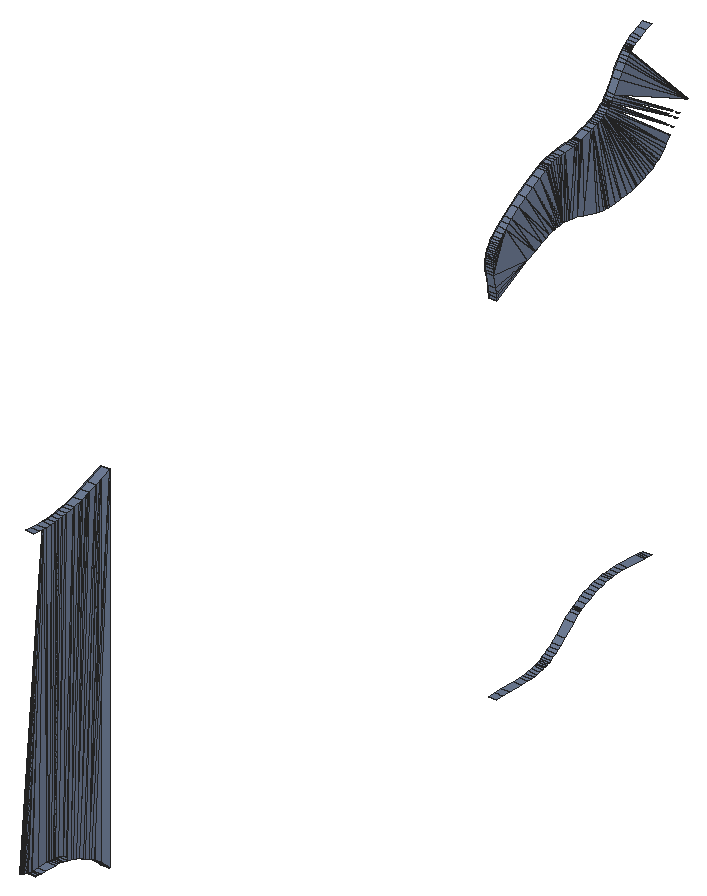
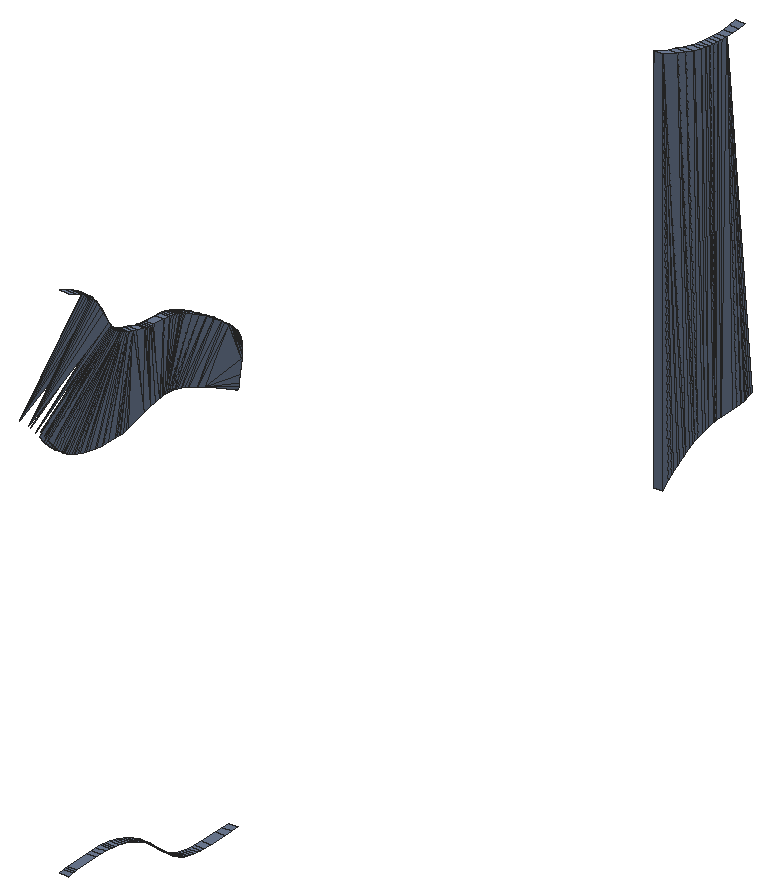
# SketchUp Ruby script. Lengths in inches.
U = 1.inch
M = Sketchup.active_model
def pt(a) = Geom::Point3d.new(a.map { |v| v * U })
def face(e, loops, mat)
  f = e.add_face(loops[0].map { |a| pt(a) })
  loops[1..].each { |l| e.add_face(l.map { |a| pt(a) }).erase! }
  f.material = f.back_material = mat if mat
  f
end
# faces: each face lists its corners as indices into pts; further lists are holes
def faces(e, pts, list, mat = nil) = list.each { |f| face(e, (f[0].is_a?(Array) ? f : [f]).map { |l| l.map { |i| pts[i] } }, mat) }
# xy, xz, yz: faces in a plane at the given z, y or x. An outline is a flat list of corners, or four numbers for a rectangle; further outlines are holes
def ring(l) = l.size == 4 ? [[l[0], l[1]], [l[2], l[1]], [l[2], l[3]], [l[0], l[3]]] : l.each_slice(2).to_a
def flat(e, list, mat, &to3) = list.each { |f| face(e, (f[0].is_a?(Array) ? f : [f]).map { |l| ring(l).map { |u, v| to3.(u, v) } }, mat) }
def xy(e, z, list, mat = nil) = flat(e, list, mat) { |x, y| [x, y, z] }
def xz(e, y, list, mat = nil) = flat(e, list, mat) { |x, z| [x, y, z] }
def yz(e, x, list, mat = nil) = flat(e, list, mat) { |y, z| [x, y, z] }
def lines(e, pts, list) = list.each { |a, b| e.add_line(pt(pts[a]), pt(pts[b])) }
# prism: a flat outline (further loops are holes) pulled along v
def prism(e, loops, v, mat = nil)
  f = face(e, loops, mat); d = Geom::Vector3d.new(v.map { |x| x * U })
  f.pushpull(f.normal.samedirection?(d) ? d.length : -d.length)
end
def box(e, o, s, mat = nil) = prism(e, [[o, [o[0] + s[0], o[1], o[2]], [o[0] + s[0], o[1] + s[1], o[2]], [o[0], o[1] + s[1], o[2]]]], [0, 0, s[2]], mat)
def at(x, y, z, deg = 0) = Geom::Transformation.translation(pt([x, y, z])) * Geom::Transformation.rotation(ORIGIN, Z_AXIS, deg.degrees)
def axes(o, x, y, z) = Geom::Transformation.new([*x, 0, *y, 0, *z, 0, *pt(o).to_a, 1])
def part(name) = M.definitions.add(name)
# library, detail: a bought-in or finely detailed component or shape, given as its bounding box
def library(name, o, s) = part(name).tap { |d| box(d.entities, o, s) }
def detail(e, o, s) = box(e.add_group.entities, o, s)
def put(e, d, t, mat = nil) = e.add_instance(d, t).tap { |i| i.material = mat if mat }
def group(e, t, mat = nil) = e.add_group.tap { |g| g.transformation = t; g.material = mat if mat }.entities
root = M.entities
M.materials.add("3D66_SU_1584934530605_002").color = [112, 126, 151]
xy(root,52,[[122.5,312.65,123.07,313.02],[122.5,313.02,123.07,313.4]],"3D66_SU_1584934530605_002")
xy(root,74.33,[[122.5,311.62,123.07,311.75],[122.5,311.75,123.07,311.88]],"3D66_SU_1584934530605_002")
xy(root,75.08,[[122.5,307.875,123.07,308.02]],"3D66_SU_1584934530605_002")
xz(root,269.95,[[122.5,53.02,123.07,77.01]],"3D66_SU_1584934530605_002")
xz(root,302.18,[[122.5,74.85,123.07,75.04],[122.5,75.04,123.07,75.14]],"3D66_SU_1584934530605_002")
yz(root,122.5,[[269.95,53.02,269.54,53.4,269.95,77.01],[269.54,53.4,269.33,53.58,269.95,77.01],[269.33,53.58,269.11,53.75,269.95,77.01],[269.11,53.75,268.89,53.9,269.95,77.01],[268.89,53.9,268.66,54.05,269.95,77.01],
  [268.66,54.05,268.43,54.2,269.95,77.01],[268.43,54.2,268.19,54.33,269.95,77.01],[268.19,54.33,267.95,54.45,268.79,76.57],[268.19,54.33,268.79,76.57,269.95,77.01],[267.95,54.45,267.72,54.5625,268.79,76.57],
  [267.72,54.5625,267.48,54.67,268.79,76.57],[267.48,54.67,267.23,54.76,268.2,76.37],[267.48,54.67,268.2,76.37,268.79,76.57],[267.23,54.76,266.98,54.85,267.6,76.18],[267.23,54.76,267.6,76.18,268.2,76.37],
  [266.98,54.85,266.71,54.93,267.6,76.18],[266.71,54.93,266.43,55,266.99,76.03],[266.71,54.93,266.99,76.03,267.6,76.18],[266.43,55,266.13,55.07,266.68,75.97],[266.43,55,266.68,75.97,266.99,76.03],
  [266.13,55.07,266.05,55.09,266.37,75.91],[266.13,55.07,266.37,75.91,266.68,75.97],[266.05,55.09,265.97,55.1,266.37,75.91],[265.97,55.1,265.79,55.12,266.05,75.87],[265.97,55.1,266.05,75.87,266.37,75.91],
  [265.79,55.12,265.61,55.13,265.72,75.84],[265.79,55.12,265.72,75.84,266.05,75.87],[265.61,55.13,265.4,75.82,265.72,75.84],[265.61,55.13,265.43,55.14,265.4,75.82],[265.43,55.14,264.64,55.15,265.06,75.81],
  [265.43,55.14,265.06,75.81,265.4,75.82],[264.64,55.15,264.24,55.16,265.06,75.81],[264.24,55.16,264.05,55.18,265.06,75.81],[264.05,55.18,263.86,55.2,265.06,75.81],[263.86,55.2,263.76,55.22,265.06,75.81],
  [263.76,55.22,263.67,55.24,265.06,75.81],[263.67,55.24,263.58,55.26,265.06,75.81],[263.58,55.26,263.49,55.28,265.06,75.81],[263.49,55.28,263.41,55.31,265.06,75.81],[263.41,55.31,263.32,55.34,265.06,75.81],
  [263.32,55.34,263.24,55.37,265.06,75.81],[263.24,55.37,263.16,55.41,265.06,75.81],[302.48,72.84,302.47,73.04,304.99,74.12],[302.47,73.04,302.45,73.24,304.99,74.12],[302.45,73.24,302.38,73.64,304.99,74.12],
  [302.38,73.64,302.22,74.45,304.99,74.12],[304.99,74.12,302.22,74.45,303.24,76.8],[304.99,74.12,303.24,76.8,305.61,74.43],[311.62,74.33,310.54,79.64,311.75,74.33],[311.62,74.33,311.49,74.35,310.54,79.64],
  [311.75,74.33,310.54,79.64,311.88,74.33],[311.88,74.33,310.54,79.64,310.83,79.73],[311.88,74.33,310.83,79.73,312.39,74.34],[312.39,74.34,310.83,79.73,310.97,79.78],[312.39,74.34,310.97,79.78,312.89,74.375],
  [311.49,74.35,311.36,74.36,310.54,79.64],[311.36,74.36,311.09,74.41,310.54,79.64],[312.89,74.375,310.97,79.78,311.11,79.84],[312.89,74.375,311.11,79.84,313.38,74.43],[311.09,74.41,310.83,74.47,310.54,79.64],
  [305.61,74.43,303.24,76.8,303.49,77],[305.61,74.43,303.49,77,303.75,77.21],[305.61,74.43,303.75,77.21,306.23,74.69],[313.38,74.43,311.11,79.84,311.24,79.9],[313.38,74.43,311.24,79.9,313.86,74.51],
  [302.22,74.45,302.2,74.65,303.01,76.6],[302.22,74.45,303.01,76.6,303.24,76.8],[310.83,74.47,309.73,74.77,310.54,79.64],[313.86,74.51,311.24,79.9,314.1,74.57],[314.1,74.57,311.24,79.9,311.375,79.97],
  [314.1,74.57,311.375,79.97,314.33,74.625],[314.33,74.625,311.375,79.97,314.56,74.6875],[302.2,74.65,302.18,74.85,302.8,76.4],[302.2,74.65,302.8,76.4,303.01,76.6],[314.56,74.6875,311.375,79.97,314.78,74.76],
  [306.23,74.69,303.75,77.21,304.33,77.6],[306.23,74.69,304.33,77.6,306.54,74.81],[314.78,74.76,311.375,79.97,315,74.84],[309.73,74.77,309.17,74.92,309.61,79.39],[309.73,74.77,309.61,79.39,310.25,79.5625],
  [309.73,74.77,310.25,79.5625,310.54,79.64],[306.54,74.81,304.33,77.6,306.84,74.9],[315,74.84,311.375,79.97,311.51,80.05],[315,74.84,311.51,80.05,315.22,74.94],[302.18,74.85,302.18,75.04,302.8,76.4],
  [306.84,74.9,304.33,77.6,304.92,77.98],[306.84,74.9,304.92,77.98,307.14,74.98],[309.17,74.92,308.88,74.98,309.27,79.32],[309.17,74.92,309.27,79.32,309.44,79.35],[309.17,74.92,309.44,79.35,309.53,79.37],
  [309.17,74.92,309.53,79.37,309.61,79.39],[315.22,74.94,311.51,80.05,315.43,75.03],[307.14,74.98,304.92,77.98,307.29,75.01],[308.88,74.98,308.6,75.03,309.1,79.3],[308.88,74.98,309.1,79.3,309.27,79.32],
  [307.29,75.01,304.92,77.98,305.51,78.32],[307.29,75.01,305.51,78.32,307.44,75.04],[308.6,75.03,308.19,79.25,308.92,79.29],[308.6,75.03,308.45,75.05,308.19,79.25],[308.6,75.03,308.92,79.29,309.1,79.3],
  [315.43,75.03,311.51,80.05,315.64,75.14],[302.18,75.04,302.18,75.14,302.625,76.2],[302.18,75.04,302.625,76.2,302.71,76.3],[302.18,75.04,302.71,76.3,302.8,76.4],[307.44,75.04,305.51,78.32,307.58,75.06],
  [308.45,75.05,308.31,75.0625,308.19,79.25],[307.58,75.06,305.51,78.32,306.07,78.62],[307.58,75.06,306.07,78.62,307.73,75.07],[308.31,75.0625,308.16,75.07,308.19,79.25],[307.73,75.07,306.07,78.62,307.875,75.08],
  [308.16,75.07,307.81,79.21,308.19,79.25],[308.16,75.07,308.02,75.08,307.81,79.21],[307.875,75.08,306.07,78.62,306.56,78.86],[307.875,75.08,306.56,78.86,306.67,78.91],[307.875,75.08,306.67,78.91,306.78,78.96],
  [307.875,75.08,306.78,78.96,306.88,79],[307.875,75.08,306.88,79,306.99,79.04],[307.875,75.08,306.99,79.04,308.02,75.08],[308.02,75.08,306.99,79.04,307.2,79.1],[308.02,75.08,307.2,79.1,307.41,79.15],
  [308.02,75.08,307.41,79.15,307.61,79.1875],[308.02,75.08,307.61,79.1875,307.81,79.21],[302.18,75.14,302.19,75.24,302.55,76.11],[302.18,75.14,302.55,76.11,302.625,76.2],[315.64,75.14,311.51,80.05,315.74,75.2],
  [315.74,75.2,311.51,80.05,315.84,75.26],[302.19,75.24,302.21,75.34,302.55,76.11],[315.84,75.26,311.51,80.05,315.93,75.33],[315.93,75.33,311.51,80.05,316.02,75.4],[302.21,75.34,302.23,75.4375,302.48,76.01],
  [302.21,75.34,302.48,76.01,302.55,76.11],[316.02,75.4,311.51,80.05,316.2,75.55],[302.23,75.4375,302.25,75.53,302.48,76.01],[302.25,75.53,302.28,75.63,302.32,75.73],[302.25,75.53,302.32,75.73,302.37,75.82],
  [302.25,75.53,302.37,75.82,302.42,75.92],[302.25,75.53,302.42,75.92,302.48,76.01],[316.2,75.55,311.51,80.05,316.36,75.71],[316.36,75.71,311.51,80.05,316.52,75.88],[316.52,75.88,311.51,80.05,316.68,76.06],
  [316.68,76.06,311.51,80.05,311.64,80.13],[316.68,76.06,311.64,80.13,311.77,80.23],[316.68,76.06,311.77,80.23,316.98,76.43],[316.98,76.43,311.77,80.23,311.9,80.33],[317.3,76.82,311.9,80.33,311.97,80.39],
  [317.3,76.82,311.97,80.39,312.03,80.45],[317.3,76.82,312.03,80.45,312.09,80.52],[317.64,77.21,312.09,80.52,312.15,80.59],[317.64,77.21,312.15,80.59,312.27,80.74],[317.82,77.41,312.27,80.74,312.38,80.9],
  [318.47,77.96,312.38,80.9,312.8,81.6],[318.47,77.96,312.8,81.6,313.02,81.97],[318.47,77.96,313.02,81.97,313.25,82.34],[318.47,77.96,313.25,82.34,313.38,82.51],[318.47,77.96,313.38,82.51,313.51,82.67],
  [318.47,77.96,313.51,82.67,313.66,82.83],[318.47,77.96,313.66,82.83,313.73,82.9]],"3D66_SU_1584934530605_002")
yz(root,123.07,[[268.66,54.05,269.95,77.01,268.43,54.2],[268.43,54.2,269.95,77.01,268.19,54.33],[268.19,54.33,268.79,76.57,267.95,54.45],[267.95,54.45,268.79,76.57,267.72,54.5625],[267.72,54.5625,268.79,76.57,267.48,54.67],
  [267.48,54.67,268.2,76.37,267.23,54.76],[267.23,54.76,267.6,76.18,266.98,54.85],[266.98,54.85,267.6,76.18,266.71,54.93],[266.71,54.93,266.99,76.03,266.43,55],[302.48,72.84,304.99,74.12,302.47,73.04],
  [302.47,73.04,304.99,74.12,302.45,73.24],[302.45,73.24,304.99,74.12,302.38,73.64],[302.38,73.64,304.99,74.12,302.22,74.45],[304.99,74.12,303.24,76.8,302.22,74.45],[304.99,74.12,305.61,74.43,303.24,76.8],
  [311.62,74.33,310.54,79.64,311.49,74.35],[311.62,74.33,311.75,74.33,310.54,79.64],[311.75,74.33,311.88,74.33,310.54,79.64],[311.88,74.33,310.83,79.73,310.54,79.64],[311.88,74.33,312.39,74.34,310.83,79.73],
  [312.39,74.34,310.97,79.78,310.83,79.73],[312.39,74.34,312.89,74.375,310.97,79.78],[311.49,74.35,310.54,79.64,311.36,74.36],[311.36,74.36,310.54,79.64,311.09,74.41],[312.89,74.375,311.11,79.84,310.97,79.78],
  [312.89,74.375,313.38,74.43,311.11,79.84],[311.09,74.41,310.54,79.64,310.83,74.47],[305.61,74.43,303.49,77,303.24,76.8],[305.61,74.43,303.75,77.21,303.49,77],[305.61,74.43,306.23,74.69,303.75,77.21],
  [313.38,74.43,311.24,79.9,311.11,79.84],[313.38,74.43,313.86,74.51,311.24,79.9],[302.22,74.45,303.01,76.6,302.2,74.65],[302.22,74.45,303.24,76.8,303.01,76.6],[310.83,74.47,310.54,79.64,309.73,74.77],
  [313.86,74.51,314.1,74.57,311.24,79.9],[314.1,74.57,311.375,79.97,311.24,79.9],[314.1,74.57,314.33,74.625,311.375,79.97],[314.33,74.625,314.56,74.6875,311.375,79.97],[302.2,74.65,302.8,76.4,302.18,74.85],
  [302.2,74.65,303.01,76.6,302.8,76.4],[314.56,74.6875,314.78,74.76,311.375,79.97],[306.23,74.69,304.33,77.6,303.75,77.21],[306.23,74.69,306.54,74.81,304.33,77.6],[314.78,74.76,315,74.84,311.375,79.97],
  [309.73,74.77,309.61,79.39,309.17,74.92],[309.73,74.77,310.25,79.5625,309.61,79.39],[309.73,74.77,310.54,79.64,310.25,79.5625],[306.54,74.81,306.84,74.9,304.33,77.6],[315,74.84,311.51,80.05,311.375,79.97],
  [315,74.84,315.22,74.94,311.51,80.05],[302.18,74.85,302.8,76.4,302.18,75.04],[306.84,74.9,304.92,77.98,304.33,77.6],[306.84,74.9,307.14,74.98,304.92,77.98],[309.17,74.92,309.27,79.32,308.88,74.98],
  [309.17,74.92,309.44,79.35,309.27,79.32],[309.17,74.92,309.53,79.37,309.44,79.35],[309.17,74.92,309.61,79.39,309.53,79.37],[315.22,74.94,315.43,75.03,311.51,80.05],[307.14,74.98,307.29,75.01,304.92,77.98],
  [308.88,74.98,309.1,79.3,308.6,75.03],[308.88,74.98,309.27,79.32,309.1,79.3],[307.29,75.01,305.51,78.32,304.92,77.98],[307.29,75.01,307.44,75.04,305.51,78.32],[308.6,75.03,308.19,79.25,308.45,75.05],
  [308.6,75.03,308.92,79.29,308.19,79.25],[308.6,75.03,309.1,79.3,308.92,79.29],[315.43,75.03,315.64,75.14,311.51,80.05],[302.18,75.04,302.625,76.2,302.18,75.14],[302.18,75.04,302.71,76.3,302.625,76.2],
  [302.18,75.04,302.8,76.4,302.71,76.3],[307.44,75.04,307.58,75.06,305.51,78.32],[308.45,75.05,308.19,79.25,308.31,75.0625],[307.58,75.06,306.07,78.62,305.51,78.32],[307.58,75.06,307.73,75.07,306.07,78.62],
  [308.31,75.0625,308.19,79.25,308.16,75.07],[307.73,75.07,307.875,75.08,306.07,78.62],[308.16,75.07,307.81,79.21,308.02,75.08],[308.16,75.07,308.19,79.25,307.81,79.21],[307.875,75.08,306.56,78.86,306.07,78.62],
  [307.875,75.08,306.67,78.91,306.56,78.86],[307.875,75.08,306.78,78.96,306.67,78.91],[307.875,75.08,306.88,79,306.78,78.96],[307.875,75.08,306.99,79.04,306.88,79],[307.875,75.08,308.02,75.08,306.99,79.04],
  [308.02,75.08,307.2,79.1,306.99,79.04],[308.02,75.08,307.41,79.15,307.2,79.1],[308.02,75.08,307.61,79.1875,307.41,79.15],[308.02,75.08,307.81,79.21,307.61,79.1875],[302.18,75.14,302.55,76.11,302.19,75.24],
  [302.18,75.14,302.625,76.2,302.55,76.11],[315.64,75.14,315.74,75.2,311.51,80.05],[315.74,75.2,315.84,75.26,311.51,80.05],[302.19,75.24,302.55,76.11,302.21,75.34],[315.84,75.26,315.93,75.33,311.51,80.05],
  [315.93,75.33,316.02,75.4,311.51,80.05],[302.21,75.34,302.48,76.01,302.23,75.4375],[302.21,75.34,302.55,76.11,302.48,76.01],[316.02,75.4,316.2,75.55,311.51,80.05],[302.23,75.4375,302.48,76.01,302.25,75.53],
  [302.25,75.53,302.32,75.73,302.28,75.63],[302.25,75.53,302.37,75.82,302.32,75.73],[302.25,75.53,302.42,75.92,302.37,75.82],[302.25,75.53,302.48,76.01,302.42,75.92],[316.2,75.55,316.36,75.71,311.51,80.05],
  [316.36,75.71,316.52,75.88,311.51,80.05],[316.52,75.88,316.68,76.06,311.51,80.05],[316.68,76.06,311.64,80.13,311.51,80.05],[316.68,76.06,311.77,80.23,311.64,80.13],[316.68,76.06,316.98,76.43,311.77,80.23],
  [316.98,76.43,311.9,80.33,311.77,80.23],[317.3,76.82,311.97,80.39,311.9,80.33],[317.3,76.82,312.03,80.45,311.97,80.39],[317.3,76.82,312.09,80.52,312.03,80.45],[317.64,77.21,312.15,80.59,312.09,80.52],
  [317.64,77.21,312.27,80.74,312.15,80.59],[317.82,77.41,312.38,80.9,312.27,80.74],[318.47,77.96,312.8,81.6,312.38,80.9],[318.47,77.96,313.02,81.97,312.8,81.6],[318.47,77.96,313.25,82.34,313.02,81.97],
  [318.47,77.96,313.38,82.51,313.25,82.34],[318.47,77.96,313.51,82.67,313.38,82.51],[318.47,77.96,313.66,82.83,313.51,82.67],[318.47,77.96,313.73,82.9,313.66,82.83]],"3D66_SU_1584934530605_002")
p = [[123.07,303,48.85],[122.5,303,48.85],[122.5,302.48,48.84],[123.07,302.48,48.84],[123.07,303.52,48.84],[122.5,303.52,48.84],
  [123.07,304.58,48.81],[122.5,304.58,48.81],[123.07,305.1,48.82],[122.5,305.1,48.82],[123.07,305.36,48.83],[122.5,305.36,48.83],
  [123.07,305.61,48.85],[122.5,305.61,48.85],[123.07,305.85,48.88],[122.5,305.85,48.88],[123.07,306.09,48.92],[122.5,306.09,48.92],
  [123.07,306.33,48.97],[122.5,306.33,48.97],[123.07,306.44,49],[122.5,306.44,49],[123.07,306.56,49.03],[122.5,306.56,49.03],
  [123.07,306.67,49.07],[122.5,306.67,49.07],[123.07,306.78,49.12],[122.5,306.78,49.12],[123.07,306.88,49.16],[122.5,306.88,49.16],
  [123.07,306.99,49.22],[122.5,306.99,49.22],[123.07,307.2,49.33],[122.5,307.2,49.33],[123.07,307.41,49.46],[122.5,307.41,49.46],
  [123.07,307.61,49.6],[122.5,307.61,49.6],[123.07,307.81,49.75],[122.5,307.81,49.75],[123.07,308.19,50.06],[122.5,308.19,50.06],
  [123.07,308.92,50.67],[122.5,308.92,50.67],[123.07,309.27,50.94],[122.5,309.27,50.94],[123.07,309.44,51.06],[122.5,309.44,51.06],
  [122.5,309.53,51.11],[123.07,309.53,51.11],[122.5,309.61,51.16],[123.07,309.61,51.16],[123.07,309.93,51.32],[122.5,309.93,51.32],
  [123.07,310.23,51.46],[122.5,310.23,51.46],[123.07,310.51,51.58],[122.5,310.51,51.58],[123.07,310.79,51.68],[122.5,310.79,51.68],
  [123.07,311.06,51.76],[122.5,311.06,51.76],[123.07,311.34,51.83],[122.5,311.34,51.83],[123.07,311.63,51.89],[122.5,311.63,51.89],
  [123.07,315.45,51.84],[122.5,315.45,51.84],[122.5,315.15,51.89],[123.07,315.15,51.89],[123.07,311.94,51.9375],[122.5,311.94,51.9375],
  [123.07,312.11,51.96],[122.5,312.11,51.96],[123.07,314.84,51.92],[122.5,314.84,51.92],[122.5,313.4,52],[123.07,313.4,52],
  [123.07,315,51.91],[122.5,315,51.91],[123.07,312.29,51.98],[122.5,312.29,51.98],[123.07,312.65,52],[122.5,312.65,52],
  [123.07,269.54,53.4],[122.5,269.54,53.4],[122.5,269.95,53.02],[123.07,269.95,53.02],[123.07,269.33,53.58],[122.5,269.33,53.58],
  [123.07,269.11,53.75],[122.5,269.11,53.75],[123.07,268.89,53.9],[122.5,268.89,53.9],[123.07,268.66,54.05],[122.5,268.66,54.05],
  [123.07,268.43,54.2],[122.5,268.43,54.2],[123.07,268.19,54.33],[122.5,268.19,54.33],[123.07,267.95,54.45],[122.5,267.95,54.45],
  [123.07,267.72,54.5625],[122.5,267.72,54.5625],[123.07,267.48,54.67],[122.5,267.48,54.67],[123.07,267.23,54.76],[122.5,267.23,54.76],
  [123.07,266.71,54.93],[122.5,266.71,54.93],[122.5,266.98,54.85],[123.07,266.98,54.85],[123.07,266.43,55],[122.5,266.43,55],
  [123.07,266.13,55.07],[122.5,266.13,55.07],[123.07,264.24,55.16],[122.5,264.24,55.16],[122.5,264.64,55.15],[123.07,264.64,55.15],
  [122.5,265.43,55.14],[123.07,265.43,55.14],[122.5,265.61,55.13],[123.07,265.61,55.13],[122.5,265.79,55.12],[123.07,265.79,55.12],
  [122.5,265.97,55.1],[123.07,265.97,55.1],[122.5,266.05,55.09],[123.07,266.05,55.09],[123.07,263.76,55.22],[122.5,263.76,55.22],
  [122.5,263.86,55.2],[123.07,263.86,55.2],[122.5,264.05,55.18],[123.07,264.05,55.18],[123.07,302.47,73.04],[122.5,302.47,73.04],
  [122.5,302.48,72.84],[123.07,302.48,72.84],[122.5,304.99,74.12],[123.07,304.99,74.12],[123.07,302.45,73.24],[122.5,302.45,73.24],
  [123.07,302.38,73.64],[122.5,302.38,73.64],[123.07,302.22,74.45],[122.5,302.22,74.45],[122.5,305.61,74.43],[123.07,305.61,74.43],
  [123.07,311.36,74.36],[122.5,311.36,74.36],[122.5,311.49,74.35],[123.07,311.49,74.35],[122.5,311.62,74.33],[123.07,311.62,74.33],
  [123.07,311.88,74.33],[122.5,311.88,74.33],[122.5,312.39,74.34],[123.07,312.39,74.34],[122.5,312.89,74.375],[123.07,312.89,74.375],
  [123.07,302.2,74.65],[122.5,302.2,74.65],[122.5,306.23,74.69],[123.07,306.23,74.69],[123.07,310.83,74.47],[122.5,310.83,74.47],
  [122.5,311.09,74.41],[123.07,311.09,74.41],[122.5,313.38,74.43],[123.07,313.38,74.43],[122.5,313.86,74.51],[123.07,313.86,74.51],
  [123.07,309.73,74.77],[122.5,309.73,74.77],[122.5,314.1,74.57],[123.07,314.1,74.57],[123.07,302.18,74.85],[122.5,302.18,74.85],
  [122.5,314.33,74.625],[123.07,314.33,74.625],[122.5,314.56,74.6875],[123.07,314.56,74.6875],[122.5,306.54,74.81],[123.07,306.54,74.81],
  [122.5,314.78,74.76],[123.07,314.78,74.76],[122.5,306.84,74.9],[123.07,306.84,74.9],[123.07,309.17,74.92],[122.5,309.17,74.92],
  [122.5,315,74.84],[123.07,315,74.84],[122.5,315.22,74.94],[123.07,315.22,74.94],[122.5,307.14,74.98],[123.07,307.14,74.98],
  [123.07,308.88,74.98],[122.5,308.88,74.98],[122.5,307.29,75.01],[123.07,307.29,75.01],[122.5,307.44,75.04],[123.07,307.44,75.04],
  [122.5,307.58,75.06],[123.07,307.58,75.06],[123.07,308.31,75.0625],[122.5,308.31,75.0625],[122.5,308.45,75.05],[123.07,308.45,75.05],
  [122.5,308.6,75.03],[123.07,308.6,75.03],[123.07,302.19,75.24],[122.5,302.19,75.24],[122.5,302.18,75.14],[123.07,302.18,75.14],
  [122.5,307.73,75.07],[123.07,307.73,75.07],[122.5,307.875,75.08],[123.07,307.875,75.08],[123.07,308.02,75.08],[122.5,308.02,75.08],
  [122.5,308.16,75.07],[123.07,308.16,75.07],[123.07,302.21,75.34],[122.5,302.21,75.34],[123.07,302.23,75.4375],[122.5,302.23,75.4375],
  [123.07,302.25,75.53],[122.5,302.25,75.53],[123.07,302.28,75.63],[122.5,302.28,75.63],[123.07,302.32,75.73],[122.5,302.32,75.73],
  [123.07,302.37,75.82],[122.5,302.37,75.82],[123.07,264.1,75.85],[122.5,264.1,75.85],[122.5,263.63,75.9],[123.07,263.63,75.9],
  [123.07,264.58,75.82],[122.5,264.58,75.82],[123.07,265.06,75.81],[122.5,265.06,75.81],[123.07,265.4,75.82],[122.5,265.4,75.82],
  [123.07,265.72,75.84],[122.5,265.72,75.84],[123.07,266.05,75.87],[122.5,266.05,75.87],[123.07,302.42,75.92],[122.5,302.42,75.92],
  [123.07,266.37,75.91],[122.5,266.37,75.91],[123.07,266.68,75.97],[122.5,266.68,75.97],[123.07,302.48,76.01],[122.5,302.48,76.01],
  [123.07,266.99,76.03],[122.5,266.99,76.03],[123.07,267.6,76.18],[122.5,267.6,76.18],[123.07,302.55,76.11],[122.5,302.55,76.11],
  [123.07,302.625,76.2],[122.5,302.625,76.2],[123.07,268.2,76.37],[122.5,268.2,76.37],[123.07,302.71,76.3],[122.5,302.71,76.3],
  [123.07,302.8,76.4],[122.5,302.8,76.4],[123.07,268.79,76.57],[122.5,268.79,76.57],[123.07,303.01,76.6],[122.5,303.01,76.6],
  [123.07,269.95,77.01],[122.5,269.95,77.01],[123.07,303.24,76.8],[122.5,303.24,76.8],[123.07,303.49,77],[122.5,303.49,77],
  [123.07,303.75,77.21],[122.5,303.75,77.21],[123.07,304.33,77.6],[122.5,304.33,77.6],[123.07,304.92,77.98],[122.5,304.92,77.98],
  [123.07,305.51,78.32],[122.5,305.51,78.32],[123.07,306.07,78.62],[122.5,306.07,78.62],[123.07,306.56,78.86],[122.5,306.56,78.86],
  [123.07,306.67,78.91],[122.5,306.67,78.91],[123.07,306.78,78.96],[122.5,306.78,78.96],[123.07,306.88,79],[122.5,306.88,79],
  [123.07,306.99,79.04],[122.5,306.99,79.04],[123.07,307.2,79.1],[122.5,307.2,79.1],[123.07,307.41,79.15],[122.5,307.41,79.15],
  [123.07,307.61,79.1875],[122.5,307.61,79.1875],[123.07,307.81,79.21],[122.5,307.81,79.21],[123.07,308.19,79.25],[122.5,308.19,79.25],
  [123.07,308.92,79.29],[122.5,308.92,79.29],[123.07,309.1,79.3],[122.5,309.1,79.3],[123.07,309.27,79.32],[122.5,309.27,79.32],
  [123.07,309.44,79.35],[122.5,309.44,79.35],[123.07,309.53,79.37],[122.5,309.53,79.37],[123.07,309.61,79.39],[122.5,309.61,79.39],
  [123.07,310.25,79.5625],[122.5,310.25,79.5625],[123.07,310.54,79.64],[122.5,310.54,79.64],[123.07,310.83,79.73],[122.5,310.83,79.73],
  [123.07,310.97,79.78],[122.5,310.97,79.78],[123.07,311.11,79.84],[122.5,311.11,79.84],[123.07,311.24,79.9],[122.5,311.24,79.9],
  [123.07,311.375,79.97],[122.5,311.375,79.97],[123.07,311.51,80.05],[122.5,311.51,80.05],[123.07,311.64,80.13],[122.5,311.64,80.13],
  [123.07,311.77,80.23],[122.5,311.77,80.23],[123.07,311.9,80.33],[122.5,311.9,80.33],[122.5,311.97,80.39],[123.07,311.97,80.39],
  [122.5,312.03,80.45],[123.07,312.03,80.45],[122.5,312.09,80.52],[123.07,312.09,80.52],[122.5,312.15,80.59],[123.07,312.15,80.59],
  [123.07,312.27,80.74],[122.5,312.27,80.74],[123.07,312.38,80.9],[122.5,312.38,80.9],[123.07,312.8,81.6],[122.5,312.8,81.6],
  [123.07,313.02,81.97],[122.5,313.02,81.97],[123.07,313.25,82.34],[122.5,313.25,82.34],[123.07,313.38,82.51],[122.5,313.38,82.51],
  [123.07,313.51,82.67],[122.5,313.51,82.67],[123.07,313.66,82.83],[122.5,313.66,82.83],[123.07,313.73,82.9],[122.5,313.73,82.9],
  [122.5,313.8125,82.97],[123.07,313.8125,82.97],[122.5,313.89,83.03],[123.07,313.89,83.03],[122.5,313.98,83.1],[123.07,313.98,83.1],
  [123.07,314.16,83.22],[122.5,314.16,83.22],[123.07,314.36,83.33],[122.5,314.36,83.33],[123.07,314.56,83.4375],[122.5,314.56,83.4375],
  [123.07,314.99,83.64],[122.5,314.99,83.64],[123.07,315.43,83.82],[122.5,315.43,83.82]]
faces(root,p,[[0,1,2,3],[4,5,1,0],[6,7,5,4],[8,9,7,6],[10,11,9,8],[12,13,11,10],[14,15,13,12],[16,17,15,14],
  [18,19,17,16],[20,21,19,18],[22,23,21,20],[24,25,23,22],[26,27,25,24],[28,29,27,26],[30,31,29,28],[32,33,31,30],
  [34,35,33,32],[36,37,35,34],[38,39,37,36],[40,41,39,38],[42,43,41,40],[44,45,43,42],[46,47,45,44],[48,47,46],
  [48,46,49],[50,48,49],[50,49,51],[52,53,50,51],[54,55,53,52],[56,57,55,54],[58,59,57,56],[60,61,59,58],
  [62,63,61,60],[64,65,63,62],[66,67,68,69],[70,71,65,64],[72,73,71,70],[74,75,76,77],[78,79,75,74],[69,68,79,78],
  [80,81,73,72],[82,83,81,80],[84,85,86,87],[88,89,85,84],[90,91,89,88],[92,93,91,90],[94,95,93,92],[96,97,95,94],
  [98,99,97,96],[100,101,99,98],[102,103,101,100],[104,105,103,102],[106,107,105,104],[108,109,110,111],[111,110,107,106],[112,113,109,108],
  [114,115,113,112],[116,117,118,119],[119,118,120,121],[121,120,122,123],[123,122,124,125],[125,124,126,127],[127,126,128,129],[129,128,115,114],
  [130,131,132,133],[133,132,134,135],[135,134,117,116],[136,137,138,139],[139,138,140,141],[142,143,137,136],[144,145,143,142],[146,147,145,144],
  [141,140,148,149],[150,151,152,153],[153,152,154,155],[156,157,158,159],[159,158,160,161],[162,163,147,146],[149,148,164,165],[166,167,168,169],
  [169,168,151,150],[161,160,170,171],[171,170,172,173],[174,175,167,166],[173,172,176,177],[178,179,163,162],[177,176,180,181],[181,180,182,183],
  [165,164,184,185],[183,182,186,187],[185,184,188,189],[190,191,175,174],[187,186,192,193],[193,192,194,195],[189,188,196,197],[198,199,191,190],
  [197,196,200,201],[201,200,202,203],[203,202,204,205],[206,207,208,209],[209,208,210,211],[211,210,199,198],[212,213,214,215],[205,204,216,217],
  [217,216,218,219],[220,221,222,223],[223,222,207,206],[224,225,213,212],[226,227,225,224],[228,229,227,226],[230,231,229,228],[232,233,231,230],
  [234,235,233,232],[236,237,238,239],[240,241,237,236],[242,243,241,240],[244,245,243,242],[246,247,245,244],[248,249,247,246],[250,251,235,234],
  [252,253,249,248],[254,255,253,252],[256,257,251,250],[258,259,255,254],[260,261,259,258],[262,263,257,256],[264,265,263,262],[266,267,261,260],
  [268,269,265,264],[270,271,269,268],[272,273,267,266],[274,275,271,270],[276,277,273,272],[278,279,275,274],[280,281,279,278],[282,283,281,280],
  [284,285,283,282],[286,287,285,284],[288,289,287,286],[290,291,289,288],[292,293,291,290],[294,295,293,292],[296,297,295,294],[298,299,297,296],
  [300,301,299,298],[302,303,301,300],[304,305,303,302],[306,307,305,304],[308,309,307,306],[310,311,309,308],[312,313,311,310],[314,315,313,312],
  [316,317,315,314],[318,319,317,316],[320,321,319,318],[322,323,321,320],[324,325,323,322],[326,327,325,324],[328,329,327,326],[330,331,329,328],
  [332,333,331,330],[334,335,333,332],[336,337,335,334],[338,339,337,336],[340,341,339,338],[342,343,341,340],[344,345,343,342],[346,345,344],
  [346,344,347],[348,346,347],[348,347,349],[350,348,349],[350,349,351],[352,350,351],[352,351,353],[354,355,352,353],
  [356,357,355,354],[358,359,357,356],[360,361,359,358],[362,363,361,360],[364,365,363,362],[366,367,365,364],[368,369,367,366],[370,371,369,368],
  [372,371,370],[372,370,373],[374,372,373],[374,373,375],[376,374,375],[376,375,377],[378,379,376,377],[380,381,379,378],
  [382,383,381,380],[384,385,383,382],[386,387,385,384]],"3D66_SU_1584934530605_002")
